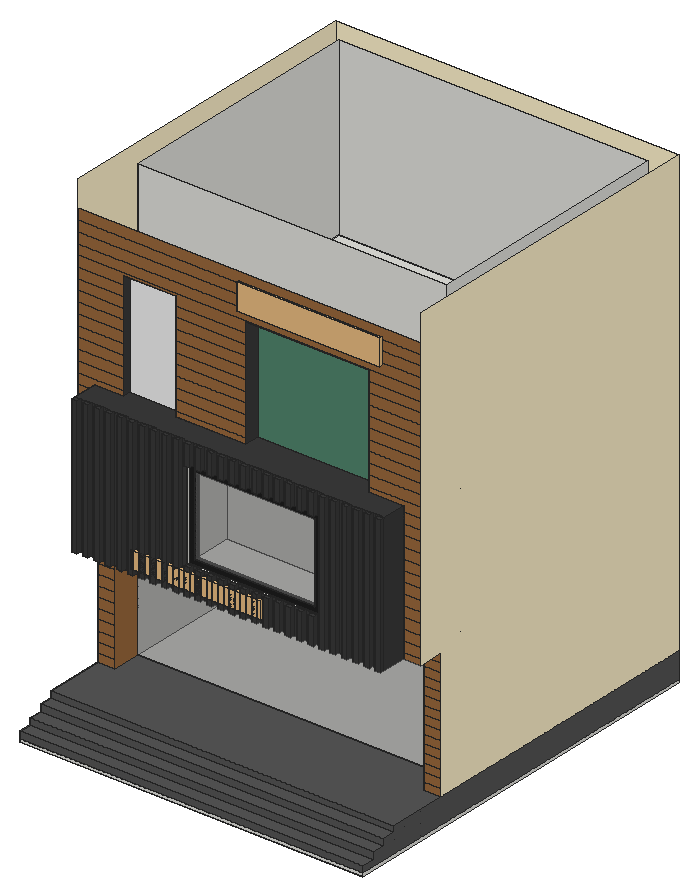
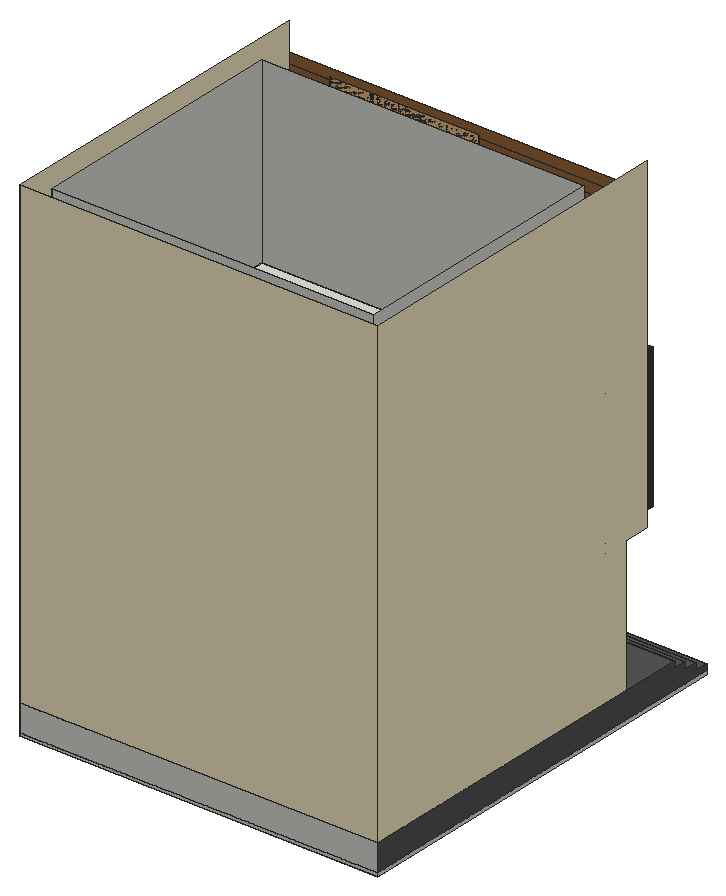
# SketchUp Ruby script. Lengths in inches.
U = 1.inch
M = Sketchup.active_model
def pt(a) = Geom::Point3d.new(a.map { |v| v * U })
def face(e, loops, mat)
  f = e.add_face(loops[0].map { |a| pt(a) })
  loops[1..].each { |l| e.add_face(l.map { |a| pt(a) }).erase! }
  f.material = f.back_material = mat if mat
  f
end
# faces: each face lists its corners as indices into pts; further lists are holes
def faces(e, pts, list, mat = nil) = list.each { |f| face(e, (f[0].is_a?(Array) ? f : [f]).map { |l| l.map { |i| pts[i] } }, mat) }
# xy, xz, yz: faces in a plane at the given z, y or x. An outline is a flat list of corners, or four numbers for a rectangle; further outlines are holes
def ring(l) = l.size == 4 ? [[l[0], l[1]], [l[2], l[1]], [l[2], l[3]], [l[0], l[3]]] : l.each_slice(2).to_a
def flat(e, list, mat, &to3) = list.each { |f| face(e, (f[0].is_a?(Array) ? f : [f]).map { |l| ring(l).map { |u, v| to3.(u, v) } }, mat) }
def xy(e, z, list, mat = nil) = flat(e, list, mat) { |x, y| [x, y, z] }
def xz(e, y, list, mat = nil) = flat(e, list, mat) { |x, z| [x, y, z] }
def yz(e, x, list, mat = nil) = flat(e, list, mat) { |y, z| [x, y, z] }
def lines(e, pts, list) = list.each { |a, b| e.add_line(pt(pts[a]), pt(pts[b])) }
# prism: a flat outline (further loops are holes) pulled along v
def prism(e, loops, v, mat = nil)
  f = face(e, loops, mat); d = Geom::Vector3d.new(v.map { |x| x * U })
  f.pushpull(f.normal.samedirection?(d) ? d.length : -d.length)
end
def box(e, o, s, mat = nil) = prism(e, [[o, [o[0] + s[0], o[1], o[2]], [o[0] + s[0], o[1] + s[1], o[2]], [o[0], o[1] + s[1], o[2]]]], [0, 0, s[2]], mat)
def at(x, y, z, deg = 0) = Geom::Transformation.translation(pt([x, y, z])) * Geom::Transformation.rotation(ORIGIN, Z_AXIS, deg.degrees)
def axes(o, x, y, z) = Geom::Transformation.new([*x, 0, *y, 0, *z, 0, *pt(o).to_a, 1])
def part(name) = M.definitions.add(name)
# library, detail: a bought-in or finely detailed component or shape, given as its bounding box
def library(name, o, s) = part(name).tap { |d| box(d.entities, o, s) }
def detail(e, o, s) = box(e.add_group.entities, o, s)
def put(e, d, t, mat = nil) = e.add_instance(d, t).tap { |i| i.material = mat if mat }
def group(e, t, mat = nil) = e.add_group.tap { |g| g.transformation = t; g.material = mat if mat }.entities
root = M.entities
M.materials.add("[Color D01]").color = [255, 242, 204]
M.materials.add("[Color M06]").color = [86, 86, 86]
M.materials.add("[Color M07]").color = [58, 58, 58]
M.materials.add("[Color M08]").color = [30, 30, 30]
M.materials.add("[Terrazzo]").color = [241, 241, 241]
M.materials.add("[Translucent Glass Gray]").color = [128, 128, 128]
M.materials["[Translucent Glass Gray]"].alpha = 0.5
M.materials.add("[Vegetation Ivy Hedera]").color = [81, 134, 109]
M.materials.add("[Wood Floor]").color = [155, 105, 61]
c1 = library("BRANDING\#1",[0.57,0,0],[181.63,23.97,4])
xy(root,4.8125,[[0,0,480,552]])
xy(root,9,[[0,0,480,18],[0,18,480,72],[0,72,480,552]])
xy(root,18.12,[[0,0,480,18]],"[Color M06]")
xy(root,27.24,[[0,18,480,36]],"[Color M06]")
xy(root,36.36,[[0,36,480,54]],"[Color M06]")
xy(root,45,[[0,135.75,0,552,480,552,480,135.75,456,135.75,456,528,24,528,24,135.75],[24,175.75,456,528]])
xy(root,45,[[0,54,480,54,480,135.75,456,135.75,456,175.75,24,175.75,24,135.75,0,135.75]],"[Color M06]")
xy(root,225,[[24,60.6875,31.22,66.5],[39.1,60.6875,46.97,66.5],[54.85,60.6875,62.72,66.5],[70.6,60.6875,78.47,66.5],[86.35,60.6875,94.22,66.5],
  [102.1,60.6875,109.97,66.5],[117.85,60.6875,125.72,66.5],[133.6,60.6875,141.47,66.5],[149.35,60.6875,157.22,66.5],[165.1,60.6875,172.97,66.5],
  [180.85,60.6875,188.72,66.5],[196.6,60.6875,204.47,66.5],[212.35,60.6875,220.22,66.5],[228.1,60.6875,235.97,66.5],[243.85,60.6875,251.72,66.5],
  [259.6,60.6875,267.47,66.5],[275.35,60.6875,283.22,66.5],[291.1,60.6875,298.97,66.5],[306.85,60.6875,314.72,66.5],[322.6,60.6875,330.47,66.5],
  [338.35,60.6875,346.22,66.5],[354.1,60.6875,361.97,66.5],[369.85,60.6875,377.72,66.5],[385.6,60.6875,393.47,66.5],[401.35,60.6875,409.22,66.5],
  [417.1,60.6875,424.97,66.5],[432.72,60.6875,440.47,66.5],[448.22,60.6875,455.97,66.5],[24,66.5,456,169.75]],"[Color M07]")
xy(root,225,[[0,100.625,24,135.75],[456,100.625,480,135.75]],"[Wood Floor]")
xy(root,237,[[24,175.75,24,528,462.0625,528,456,175.75]])
xy(root,243,[[24,175.75,456,175.75,462.0625,528,24,528]])
xy(root,262.33,[[180.64,66.5,367.39,136.3125]])
xy(root,262.33,[[180.85,60.6875,188.72,66.5],[196.6,60.6875,204.47,66.5],[212.35,60.6875,220.22,66.5],[228.1,60.6875,235.97,66.5],[243.85,60.6875,251.72,66.5],
  [259.6,60.6875,267.47,66.5],[275.35,60.6875,283.22,66.5],[291.1,60.6875,298.97,66.5],[306.85,60.6875,314.72,66.5],[322.6,60.6875,330.47,66.5],
  [338.35,60.6875,346.22,66.5],[354.1,60.6875,361.97,66.5]],"[Color M07]")
xy(root,387.89,[[180.64,66.5,367.39,136.3125]])
xy(root,387.89,[[180.85,60.6875,188.72,66.5],[196.6,60.6875,204.47,66.5],[212.35,60.6875,220.22,66.5],[228.1,60.6875,235.97,66.5],[243.85,60.6875,251.72,66.5],
  [259.6,60.6875,267.47,66.5],[275.35,60.6875,283.22,66.5],[291.1,60.6875,298.97,66.5],[306.85,60.6875,314.72,66.5],[322.6,60.6875,330.47,66.5],
  [338.35,60.6875,346.22,66.5],[354.1,60.6875,361.97,66.5]],"[Color M07]")
xy(root,411,[[24,175.75,456,528]])
xy(root,417,[[24,100.625,65.03,100.625,65.03,111.375,137.72,111.375,137.72,100.625,235.41,100.625,235.41,121.375,407.34,121.375,407.34,100.625,456,100.625,456,169.75,24,169.75],[24,175.75,456,528]])
xy(root,417,[[24,60.6875,31.22,66.5],[39.1,60.6875,46.97,66.5],[54.85,60.6875,62.72,66.5],[70.6,60.6875,78.47,66.5],[86.35,60.6875,94.22,66.5],
  [102.1,60.6875,109.97,66.5],[117.85,60.6875,125.72,66.5],[133.6,60.6875,141.47,66.5],[149.35,60.6875,157.22,66.5],[165.1,60.6875,172.97,66.5],
  [180.85,60.6875,188.72,66.5],[196.6,60.6875,204.47,66.5],[212.35,60.6875,220.22,66.5],[228.1,60.6875,235.97,66.5],[243.85,60.6875,251.72,66.5],
  [259.6,60.6875,267.47,66.5],[275.35,60.6875,283.22,66.5],[291.1,60.6875,298.97,66.5],[306.85,60.6875,314.72,66.5],[322.6,60.6875,330.47,66.5],
  [338.35,60.6875,346.22,66.5],[354.1,60.6875,361.97,66.5],[369.85,60.6875,377.72,66.5],[385.6,60.6875,393.47,66.5],[401.35,60.6875,409.22,66.5],
  [417.1,60.6875,424.97,66.5],[432.72,60.6875,440.47,66.5],[448.22,60.6875,455.97,66.5],[24,66.5,456,66.5,456,100.625,407.34,100.625,407.34,121.375,235.41,121.375,235.41,100.625,137.72,100.625,137.72,111.375,65.03,111.375,65.03,100.625,24,100.625]],"[Color M07]")
xy(root,568.1875,[[65.03,100.625,137.72,111.375]],"[Color M07]")
xy(root,570.0625,[[235.41,100.625,407.34,121.375]],"[Color M07]")
xz(root,0,[[0,4.8125,480,9]])
xz(root,0,[[0,9,480,18.12]],"[Color M06]")
xz(root,18,[[0,18.12,480,27.24]],"[Color M06]")
xz(root,36,[[0,27.24,480,36.36]],"[Color M06]")
xz(root,54,[[0,36.36,480,45]],"[Color M06]")
xz(root,60.6875,[[24,225,31.22,417],[39.1,225,46.97,417],[54.85,225,62.72,417],[70.6,225,78.47,417],[86.35,225,94.22,417],
  [102.1,225,109.97,417],[117.85,225,125.72,417],[133.6,225,141.47,417],[149.35,225,157.22,417],[165.1,225,172.97,417],
  [180.85,225,188.72,262.33],[196.6,225,204.47,262.33],[212.35,225,220.22,262.33],[228.1,225,235.97,262.33],[243.85,225,251.72,262.33],
  [259.6,225,267.47,262.33],[275.35,225,283.22,262.33],[291.1,225,298.97,262.33],[306.85,225,314.72,262.33],[322.6,225,330.47,262.33],
  [338.35,225,346.22,262.33],[354.1,225,361.97,262.33],[369.85,225,377.72,417],[385.6,225,393.47,417],[401.35,225,409.22,417],
  [417.1,225,424.97,417],[432.72,225,440.47,417],[448.22,225,455.97,417],[180.85,387.89,188.72,417],[196.6,387.89,204.47,417],
  [212.35,387.89,220.22,417],[228.1,387.89,235.97,417],[243.85,387.89,251.72,417],[259.6,387.89,267.47,417],[275.35,387.89,283.22,417],
  [291.1,387.89,298.97,417],[306.85,387.89,314.72,417],[322.6,387.89,330.47,417],[338.35,387.89,346.22,417],[354.1,387.89,361.97,417]],"[Color M07]")
xz(root,66.5,[[455.97,225,456,417]])
xz(root,66.5,[[24,225,31.22,417],[31.22,225,39.1,417],[39.1,225,46.97,417],[46.97,225,54.85,417],[54.85,225,62.72,417],
  [62.72,225,70.6,417],[70.6,225,78.47,417],[78.47,225,86.35,417],[86.35,225,94.22,417],[94.22,225,102.1,417],
  [102.1,225,109.97,417],[109.97,225,117.85,417],[117.85,225,125.72,417],[125.72,225,133.6,417],[133.6,225,141.47,417],
  [141.47,225,149.35,417],[149.35,225,157.22,417],[157.22,225,165.1,417],[165.1,225,172.97,417],[172.97,225,180.85,225,180.85,262.33,180.64,262.33,180.64,387.89,180.85,387.89,180.85,417,172.97,417],
  [180.85,225,188.72,262.33],[188.72,225,196.6,262.33],[196.6,225,204.47,262.33],[204.47,225,212.35,262.33],[212.35,225,220.22,262.33],
  [220.22,225,228.1,262.33],[228.1,225,235.97,262.33],[235.97,225,243.85,262.33],[243.85,225,251.72,262.33],[251.72,225,259.6,262.33],
  [259.6,225,267.47,262.33],[267.47,225,275.35,262.33],[275.35,225,283.22,262.33],[283.22,225,291.1,262.33],[291.1,225,298.97,262.33],
  [298.97,225,306.85,262.33],[306.85,225,314.72,262.33],[314.72,225,322.6,262.33],[322.6,225,330.47,262.33],[330.47,225,338.35,262.33],
  [338.35,225,346.22,262.33],[346.22,225,354.1,262.33],[354.1,225,361.97,262.33],[361.97,225,369.85,225,369.85,417,361.97,417,361.97,387.89,367.39,387.89,367.39,262.33,361.97,262.33],[369.85,225,377.72,417],
  [377.72,225,385.6,417],[385.6,225,393.47,417],[393.47,225,401.35,417],[401.35,225,409.22,417],[409.22,225,417.1,417],
  [417.1,225,424.97,417],[424.97,225,432.72,417],[432.72,225,440.47,417],[440.47,225,448.22,417],[448.22,225,455.97,417],
  [180.85,387.89,188.72,417],[188.72,387.89,196.6,417],[196.6,387.89,204.47,417],[204.47,387.89,212.35,417],[212.35,387.89,220.22,417],
  [220.22,387.89,228.1,417],[228.1,387.89,235.97,417],[235.97,387.89,243.85,417],[243.85,387.89,251.72,417],[251.72,387.89,259.6,417],
  [259.6,387.89,267.47,417],[267.47,387.89,275.35,417],[275.35,387.89,283.22,417],[283.22,387.89,291.1,417],[291.1,387.89,298.97,417],
  [298.97,387.89,306.85,417],[306.85,387.89,314.72,417],[314.72,387.89,322.6,417],[322.6,387.89,330.47,417],[330.47,387.89,338.35,417],
  [338.35,387.89,346.22,417],[346.22,387.89,354.1,417],[354.1,387.89,361.97,417]],"[Color M07]")
xz(root,100.625,[[0,225,24,232.9],[456,225,480,232.9],[0,232.9,24,247.58],[456,232.9,480,247.58],[0,247.58,24,262.27],
  [456,247.58,480,262.27],[0,262.27,24,276.96],[456,262.27,480,276.96],[0,276.96,24,291.65],[456,276.96,480,291.65],
  [0,291.65,24,306.33],[456,291.65,480,306.33],[0,306.33,24,321.02],[456,306.33,480,321.02],[0,321.02,24,335.71],
  [456,321.02,480,335.71],[0,335.71,24,350.4],[456,335.71,480,350.4],[0,350.4,24,365.08],[456,350.4,480,365.08],
  [0,365.08,24,379.77],[456,365.08,480,379.77],[0,379.77,24,394.46],[456,379.77,480,394.46],[0,394.46,24,409.15],
  [456,394.46,480,409.15],[0,409.15,24,409.15,24,417,65.03,417,65.03,423.83,0,423.83],[456,409.15,480,409.15,480,423.83,407.34,423.83,407.34,417,456,417],[137.72,417,235.41,423.83],[0,423.83,65.03,438.52],
  [137.72,423.83,235.41,438.52],[407.34,423.83,480,438.52],[0,438.52,65.03,453.21],[137.72,438.52,235.41,453.21],[407.34,438.52,480,453.21],
  [0,453.21,65.03,467.9],[137.72,453.21,235.41,467.9],[407.34,453.21,480,467.9],[0,467.9,65.03,482.58],[137.72,467.9,235.41,482.58],
  [407.34,467.9,480,482.58],[0,482.58,65.03,497.27],[137.72,482.58,235.41,497.27],[407.34,482.58,480,497.27],[0,497.27,65.03,511.96],
  [137.72,497.27,235.41,511.96],[407.34,497.27,480,511.96],[0,511.96,65.03,526.65],[137.72,511.96,235.41,526.65],[407.34,511.96,480,526.65],
  [0,526.65,65.03,541.33],[137.72,526.65,235.41,541.33],[407.34,526.65,480,541.33],[0,541.33,65.03,556.02],[137.72,541.33,235.41,556.02],
  [407.34,541.33,480,556.02],[0,556.02,65.03,556.02,65.03,568.1875,137.72,568.1875,137.72,556.02,235.41,556.02,235.41,570.0625,407.34,570.0625,407.34,556.02,480,556.02,480,570.71,0,570.71],[0,570.71,480,585.4],[0,585.4,480,600.08],[0,600.08,480,614.77],
  [0,614.77,480,629.46]],"[Wood Floor]")
xz(root,111.375,[[65.03,417,137.72,568.1875]],"[Terrazzo]")
xz(root,121.375,[[235.41,417,407.34,570.0625]],"[Vegetation Ivy Hedera]")
xz(root,135.75,[[0,45,24,56.29],[456,45,480,55.32],[456,55.32,480,67.25],[0,56.29,24,70.48],[456,67.25,480,79.19],
  [0,70.48,24,84.66],[456,79.19,480,91.13],[0,84.66,24,98.85],[456,91.13,480,103.25],[0,98.85,24,113.04],
  [456,103.25,480,115.38],[0,113.04,24,127.23],[456,115.38,480,127.5],[0,127.23,24,141.41],[456,127.5,480,139.63],
  [456,139.63,480,151.75],[0,141.41,24,155.6],[456,151.75,480,163.88],[0,155.6,24,169.79],[456,163.88,480,176],
  [0,169.79,24,183.98],[456,176,480,188.13],[0,183.98,24,198.16],[456,188.13,480,200.25],[0,198.16,24,212.35],
  [456,200.25,480,212.38],[0,212.35,24,225],[456,212.38,480,225]],"[Wood Floor]")
xz(root,136.3125,[[180.64,262.33,367.39,387.89]])
xz(root,169.75,[[24,225,456,237],[24,237,456,417]])
xz(root,175.75,[[24,237,456,243],[24,243,456,411],[24,411,456,417],[24,417,456,660.9375]])
xz(root,175.75,[[24,45,456,237]],"[Translucent Glass Gray]")
xz(root,528,[[24,45,456,45,461.68,225,24,225],[456,45,462.0625,225,461.68,225],[24,225,461.68,225,462.0625,237,24,237],[461.68,225,462.0625,225,462.0625,237],[24,237,462.0625,243],
  [24,243,462.0625,243,456,411,24,411],[24,411,456,417],[24,417,456,660.9375]])
xz(root,552,[[0,4.8125,480,9],[0,9,480,45]])
xz(root,552,[[0,45,480,666.9375]],"[Color D01]")
yz(root,0,[[0,4.8125,552,9]])
yz(root,0,[[135.75,45,135.75,225,100.625,225,100.625,666.9375,552,666.9375,552,45]],"[Color D01]")
yz(root,0,[[0,9,0,18.12,18,18.12,18,27.24,36,27.24,36,36.36,54,36.36,54,45,552,45,552,9]],"[Color M06]")
yz(root,24,[[175.75,45,528,225],[100.625,225,169.75,237],[175.75,225,528,237],[100.625,237,169.75,417],[175.75,237,186.125,243],
  [186.125,237,195.0625,243],[195.0625,237,528,243],[175.75,243,528,411],[175.75,411,210.65,417],[210.65,411,294.71,417],
  [294.71,411,528,417],[175.75,417,528,660.9375]])
yz(root,24,[[60.6875,225,66.5,417],[66.5,225,100.625,417]],"[Color M07]")
yz(root,24,[[135.75,45,175.75,225]],"[Wood Floor]")
yz(root,31.22,[[60.6875,225,66.5,417]],"[Color M07]")
yz(root,39.1,[[60.6875,225,66.5,417]],"[Color M07]")
yz(root,46.97,[[60.6875,225,66.5,417]],"[Color M07]")
yz(root,54.85,[[60.6875,225,66.5,417]],"[Color M07]")
yz(root,62.72,[[60.6875,225,66.5,417]],"[Color M07]")
yz(root,65.03,[[100.625,417,111.375,568.1875]],"[Color M07]")
yz(root,70.6,[[60.6875,225,66.5,417]],"[Color M07]")
yz(root,78.47,[[60.6875,225,66.5,417]],"[Color M07]")
yz(root,86.35,[[60.6875,225,66.5,417]],"[Color M07]")
yz(root,94.22,[[60.6875,225,66.5,417]],"[Color M07]")
yz(root,102.1,[[60.6875,225,66.5,417]],"[Color M07]")
yz(root,109.97,[[60.6875,225,66.5,417]],"[Color M07]")
yz(root,117.85,[[60.6875,225,66.5,417]],"[Color M07]")
yz(root,125.72,[[60.6875,225,66.5,417]],"[Color M07]")
yz(root,133.6,[[60.6875,225,66.5,417]],"[Color M07]")
yz(root,137.72,[[100.625,417,111.375,568.1875]],"[Color M07]")
yz(root,141.47,[[60.6875,225,66.5,417]],"[Color M07]")
yz(root,149.35,[[60.6875,225,66.5,417]],"[Color M07]")
yz(root,157.22,[[60.6875,225,66.5,417]],"[Color M07]")
yz(root,165.1,[[60.6875,225,66.5,417]],"[Color M07]")
yz(root,172.97,[[60.6875,225,66.5,417]],"[Color M07]")
yz(root,180.64,[[66.5,262.33,136.3125,387.89]])
yz(root,180.85,[[60.6875,225,66.5,262.33],[60.6875,387.89,66.5,417]],"[Color M07]")
yz(root,188.72,[[60.6875,225,66.5,262.33],[60.6875,387.89,66.5,417]],"[Color M07]")
yz(root,196.6,[[60.6875,225,66.5,262.33],[60.6875,387.89,66.5,417]],"[Color M07]")
yz(root,204.47,[[60.6875,225,66.5,262.33],[60.6875,387.89,66.5,417]],"[Color M07]")
yz(root,212.35,[[60.6875,225,66.5,262.33],[60.6875,387.89,66.5,417]],"[Color M07]")
yz(root,220.22,[[60.6875,225,66.5,262.33],[60.6875,387.89,66.5,417]],"[Color M07]")
yz(root,228.1,[[60.6875,225,66.5,262.33],[60.6875,387.89,66.5,417]],"[Color M07]")
yz(root,235.41,[[100.625,417,121.375,570.0625]],"[Color M07]")
yz(root,235.97,[[60.6875,225,66.5,262.33],[60.6875,387.89,66.5,417]],"[Color M07]")
yz(root,243.85,[[60.6875,225,66.5,262.33],[60.6875,387.89,66.5,417]],"[Color M07]")
yz(root,251.72,[[60.6875,225,66.5,262.33],[60.6875,387.89,66.5,417]],"[Color M07]")
yz(root,259.6,[[60.6875,225,66.5,262.33],[60.6875,387.89,66.5,417]],"[Color M07]")
yz(root,267.47,[[60.6875,225,66.5,262.33],[60.6875,387.89,66.5,417]],"[Color M07]")
yz(root,275.35,[[60.6875,225,66.5,262.33],[60.6875,387.89,66.5,417]],"[Color M07]")
yz(root,283.22,[[60.6875,225,66.5,262.33],[60.6875,387.89,66.5,417]],"[Color M07]")
yz(root,291.1,[[60.6875,225,66.5,262.33],[60.6875,387.89,66.5,417]],"[Color M07]")
yz(root,298.97,[[60.6875,225,66.5,262.33],[60.6875,387.89,66.5,417]],"[Color M07]")
yz(root,306.85,[[60.6875,225,66.5,262.33],[60.6875,387.89,66.5,417]],"[Color M07]")
yz(root,314.72,[[60.6875,225,66.5,262.33],[60.6875,387.89,66.5,417]],"[Color M07]")
yz(root,322.6,[[60.6875,225,66.5,262.33],[60.6875,387.89,66.5,417]],"[Color M07]")
yz(root,330.47,[[60.6875,225,66.5,262.33],[60.6875,387.89,66.5,417]],"[Color M07]")
yz(root,338.35,[[60.6875,225,66.5,262.33],[60.6875,387.89,66.5,417]],"[Color M07]")
yz(root,346.22,[[60.6875,225,66.5,262.33],[60.6875,387.89,66.5,417]],"[Color M07]")
yz(root,354.1,[[60.6875,225,66.5,262.33],[60.6875,387.89,66.5,417]],"[Color M07]")
yz(root,361.97,[[60.6875,225,66.5,262.33],[60.6875,387.89,66.5,417]],"[Color M07]")
yz(root,367.39,[[66.5,262.33,136.3125,387.89]])
yz(root,369.85,[[60.6875,225,66.5,417]],"[Color M07]")
yz(root,377.72,[[60.6875,225,66.5,417]],"[Color M07]")
yz(root,385.6,[[60.6875,225,66.5,417]],"[Color M07]")
yz(root,393.47,[[60.6875,225,66.5,417]],"[Color M07]")
yz(root,401.35,[[60.6875,225,66.5,417]],"[Color M07]")
yz(root,407.34,[[100.625,417,121.375,570.0625]],"[Color M07]")
yz(root,409.22,[[60.6875,225,66.5,417]],"[Color M07]")
yz(root,417.1,[[60.6875,225,66.5,417]],"[Color M07]")
yz(root,424.97,[[60.6875,225,66.5,417]],"[Color M07]")
yz(root,432.72,[[60.6875,225,66.5,417]],"[Color M07]")
yz(root,440.47,[[60.6875,225,66.5,417]],"[Color M07]")
yz(root,448.22,[[60.6875,225,66.5,417]],"[Color M07]")
yz(root,455.97,[[60.6875,225,66.5,417]],"[Color M07]")
yz(root,456,[[100.625,225,169.75,237],[100.625,237,169.75,417],[175.75,243,175.75,411,528,411],[175.75,411,528,417],[175.75,417,528,660.9375]])
yz(root,456,[[66.5,225,100.625,417]],"[Color M07]")
yz(root,456,[[135.75,45,175.75,225]],"[Wood Floor]")
yz(root,480,[[0,4.8125,552,9]])
yz(root,480,[[135.75,45,552,45,552,666.9375,100.625,666.9375,100.625,225,135.75,225]],"[Color D01]")
yz(root,480,[[0,9,552,9,552,45,54,45,54,36.36,36,36.36,36,27.24,18,27.24,18,18.12,0,18.12]],"[Color M06]")
p = [[456,175.75,237],[462.0625,528,237],[456,175.75,45],[456,175.75,225],[456,528,45],[461.68,528,225],
  [456,175.75,243],[462.0625,528,243],[456,528,411],[24,169.75,225],[0,169.75,225],[24,169.75,237],
  [0,169.75,237],[456,169.75,237],[480,169.75,237],[24,169.75,417],[0,169.75,417],[456,169.75,417],
  [480,169.75,417],[24,100.625,409.15],[456,100.625,409.15],[24,100.625,394.46],[456,100.625,394.46],[24,100.625,247.58],
  [456,100.625,247.58],[24,100.625,232.9],[456,100.625,232.9],[0,100.625,41.96],[480,100.625,41.96],[0,100.625,27.27],
  [480,100.625,27.27],[0,100.625,12.58],[480,100.625,12.58],[0,135.75,42.1],[24,135.75,42.1],[0,135.75,27.91],
  [24,135.75,27.91],[0,135.75,13.73],[24,135.75,13.73],[180.85,66.5,387.89],[180.85,66.5,262.33],[0,54,27.24],
  [480,54,27.24],[0,72,36.36],[480,72,36.36]]
faces(root,p,[[0,1,2,3],[4,2,1,5],[6,7,1,0],[7,6,8]])
lines(root,p,[[9,10],[11,12],[13,14],[15,16],[17,18],[19,20],[21,22],[23,24],[25,26],[27,28],[29,30],[31,32],
  [33,34],[35,36],[37,38],[39,40],[41,42],[43,44]])
put(root,c1,axes([106.375,64.6875,232.86],[1,0,0],[0,0,1],[0,-1,0]))
g1 = group(root,at(178.53,69.72,259.82))
xy(g1,0,[[0,0,188.86,5.97]],"[Color M08]")
xy(g1,8.82,[[10.57,0,178.28,1.72],[10.57,1.72,178.28,5.97]],"[Color M08]")
xy(g1,119.26,[[10.57,0,178.28,1.72],[10.57,1.72,178.28,5.97]],"[Color M08]")
xy(g1,128.07,[[0,0,188.86,5.97]],"[Color M08]")
xz(g1,0,[[[0,0,188.86,128.07],[10.57,8.82,178.28,119.26]]],"[Color M08]")
xz(g1,1.72,[[10.57,8.82,178.28,119.26]],"[Translucent Glass Gray]")
xz(g1,5.97,[[[0,0,188.86,128.07],[10.57,8.82,178.28,119.26]]],"[Color M08]")
yz(g1,0,[[0,0,5.97,128.07]],"[Color M08]")
yz(g1,10.57,[[0,8.82,1.72,119.26],[1.72,8.82,5.97,119.26]],"[Color M08]")
yz(g1,178.28,[[0,8.82,1.72,119.26],[1.72,8.82,5.97,119.26]],"[Color M08]")
yz(g1,188.86,[[0,0,5.97,128.07]],"[Color M08]")
put(root,c1,axes([225.14,100.625,582.12],[1.1,0,0],[0,0,1.5],[0,-1,0]))
